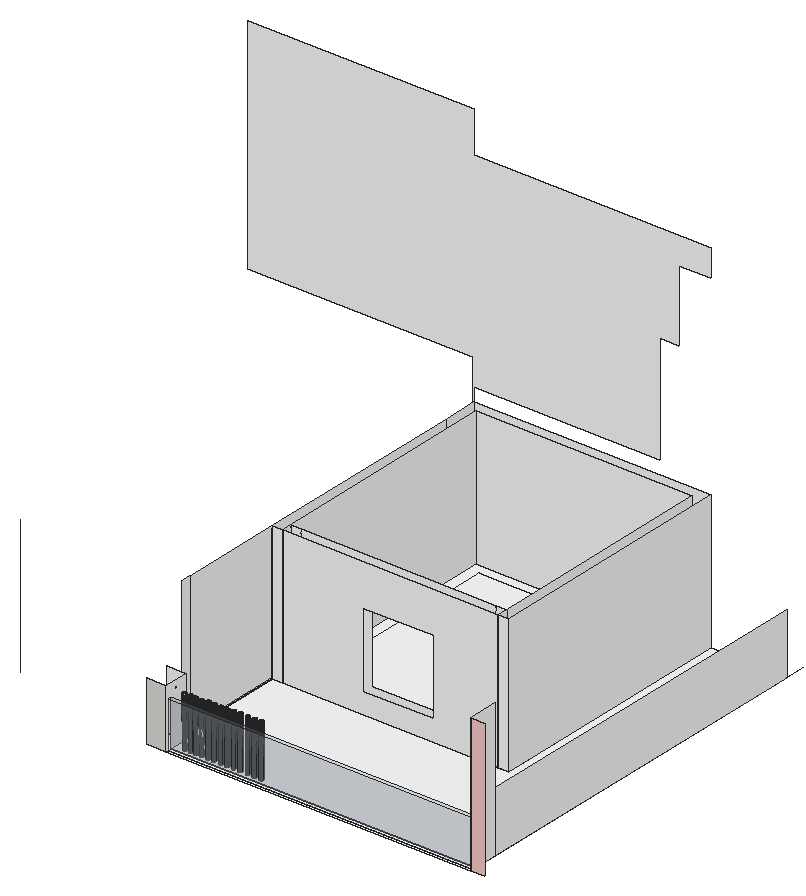
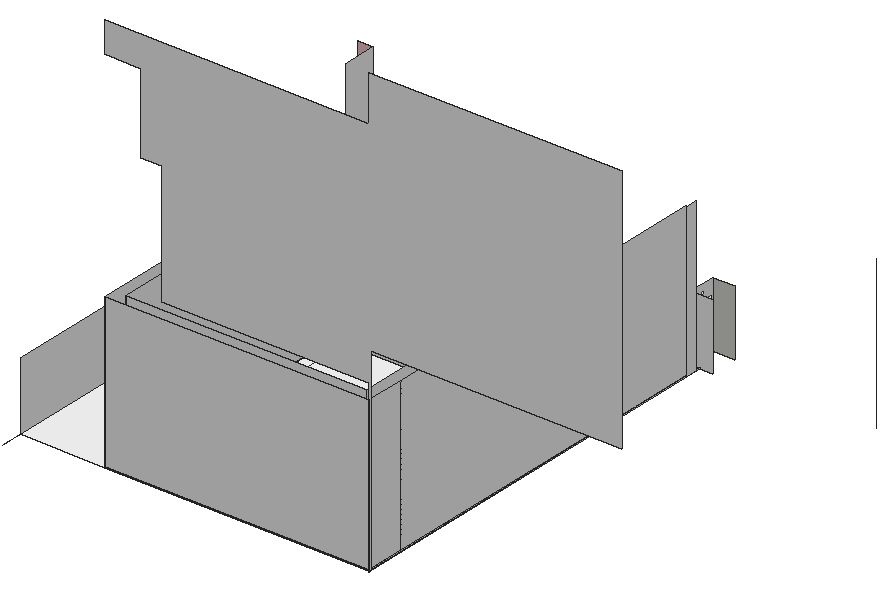
# SketchUp Ruby script. Lengths in inches.
U = 1.inch
M = Sketchup.active_model
def pt(a) = Geom::Point3d.new(a.map { |v| v * U })
def face(e, loops, mat)
  f = e.add_face(loops[0].map { |a| pt(a) })
  loops[1..].each { |l| e.add_face(l.map { |a| pt(a) }).erase! }
  f.material = f.back_material = mat if mat
  f
end
# faces: each face lists its corners as indices into pts; further lists are holes
def faces(e, pts, list, mat = nil) = list.each { |f| face(e, (f[0].is_a?(Array) ? f : [f]).map { |l| l.map { |i| pts[i] } }, mat) }
# xy, xz, yz: faces in a plane at the given z, y or x. An outline is a flat list of corners, or four numbers for a rectangle; further outlines are holes
def ring(l) = l.size == 4 ? [[l[0], l[1]], [l[2], l[1]], [l[2], l[3]], [l[0], l[3]]] : l.each_slice(2).to_a
def flat(e, list, mat, &to3) = list.each { |f| face(e, (f[0].is_a?(Array) ? f : [f]).map { |l| ring(l).map { |u, v| to3.(u, v) } }, mat) }
def xy(e, z, list, mat = nil) = flat(e, list, mat) { |x, y| [x, y, z] }
def xz(e, y, list, mat = nil) = flat(e, list, mat) { |x, z| [x, y, z] }
def yz(e, x, list, mat = nil) = flat(e, list, mat) { |y, z| [x, y, z] }
def lines(e, pts, list) = list.each { |a, b| e.add_line(pt(pts[a]), pt(pts[b])) }
# prism: a flat outline (further loops are holes) pulled along v
def prism(e, loops, v, mat = nil)
  f = face(e, loops, mat); d = Geom::Vector3d.new(v.map { |x| x * U })
  f.pushpull(f.normal.samedirection?(d) ? d.length : -d.length)
end
def box(e, o, s, mat = nil) = prism(e, [[o, [o[0] + s[0], o[1], o[2]], [o[0] + s[0], o[1] + s[1], o[2]], [o[0], o[1] + s[1], o[2]]]], [0, 0, s[2]], mat)
def at(x, y, z, deg = 0) = Geom::Transformation.translation(pt([x, y, z])) * Geom::Transformation.rotation(ORIGIN, Z_AXIS, deg.degrees)
def axes(o, x, y, z) = Geom::Transformation.new([*x, 0, *y, 0, *z, 0, *pt(o).to_a, 1])
def part(name) = M.definitions.add(name)
# library, detail: a bought-in or finely detailed component or shape, given as its bounding box
def library(name, o, s) = part(name).tap { |d| box(d.entities, o, s) }
def detail(e, o, s) = box(e.add_group.entities, o, s)
def put(e, d, t, mat = nil) = e.add_instance(d, t).tap { |i| i.material = mat if mat }
def group(e, t, mat = nil) = e.add_group.tap { |g| g.transformation = t; g.material = mat if mat }.entities
root = M.entities
M.materials.add("A01_Blush_Petal").color = [255, 204, 204]
M.materials.add("Glass_Basic_01").color = [161, 173, 186]
M.materials["Glass_Basic_01"].alpha = 0.25
M.materials.add("M00_Soft_Cloud").color = [255, 255, 255]
xy(root,264,[[205.78,136.44,472.6,138.3],[[205.78,141.64,472.6,141.64,472.6,482.39,405.98,482.39,405.98,261.09,199,261.09,199,157.97,205.78,157.97],[280.99,145.24,280.58,145.29,280.19,145.45,279.86,145.7,279.6,146.03,279.45,146.42,279.39,146.83,279.45,147.25,279.6,147.63,279.86,147.96,280.19,148.22,280.58,148.38,280.99,148.43,281.4,148.38,281.79,148.22,282.12,147.96,282.37,147.63,282.53,147.25,282.59,146.83,282.53,146.42,282.37,146.03,282.12,145.7,281.79,145.45,281.4,145.29],[256.81,145.24,256.39,145.29,256.01,145.45,255.68,145.7,255.42,146.03,255.26,146.42,255.21,146.83,255.26,147.25,255.42,147.63,255.68,147.96,256.01,148.22,256.39,148.38,256.81,148.43,257.22,148.38,257.61,148.22,257.9375,147.96,258.19,147.63,258.35,147.25,258.41,146.83,258.35,146.42,258.19,146.03,257.9375,145.7,257.61,145.45,257.22,145.29],[251.01,145.24,250.59,145.29,250.21,145.45,249.875,145.7,249.62,146.03,249.46,146.42,249.41,146.83,249.46,147.25,249.62,147.63,249.875,147.96,250.21,148.22,250.59,148.38,251.01,148.43,251.42,148.38,251.8,148.22,252.14,147.96,252.39,147.63,252.55,147.25,252.6,146.83,252.55,146.42,252.39,146.03,252.14,145.7,251.8,145.45,251.42,145.29],[245.47,145.24,245.06,145.29,244.67,145.45,244.34,145.7,244.09,146.03,243.93,146.42,243.87,146.83,243.93,147.25,244.09,147.63,244.34,147.96,244.67,148.22,245.06,148.38,245.47,148.43,245.88,148.38,246.27,148.22,246.6,147.96,246.85,147.63,247.01,147.25,247.07,146.83,247.01,146.42,246.85,146.03,246.6,145.7,246.27,145.45,245.88,145.29],[239.53,145.24,239.12,145.29,238.73,145.45,238.4,145.7,238.15,146.03,237.99,146.42,237.9375,146.83,237.99,147.25,238.15,147.63,238.4,147.96,238.73,148.22,239.12,148.38,239.53,148.43,239.95,148.38,240.33,148.22,240.66,147.96,240.92,147.63,241.08,147.25,241.13,146.83,241.08,146.42,240.92,146.03,240.66,145.7,240.33,145.45,239.95,145.29],[268.95,145.24,268.54,145.29,268.15,145.45,267.82,145.7,267.57,146.03,267.41,146.42,267.35,146.83,267.41,147.25,267.57,147.63,267.82,147.96,268.15,148.22,268.54,148.38,268.95,148.43,269.36,148.38,269.75,148.22,270.08,147.96,270.33,147.63,270.49,147.25,270.55,146.83,270.49,146.42,270.33,146.03,270.08,145.7,269.75,145.45,269.36,145.29],[262.56,145.24,262.15,145.29,261.77,145.45,261.43,145.7,261.18,146.03,261.02,146.42,260.97,146.83,261.02,147.25,261.18,147.63,261.43,147.96,261.77,148.22,262.15,148.38,262.56,148.43,262.98,148.38,263.36,148.22,263.69,147.96,263.95,147.63,264.11,147.25,264.16,146.83,264.11,146.42,263.95,146.03,263.69,145.7,263.36,145.45,262.98,145.29],[229.02,145.24,228.61,145.29,228.22,145.45,227.89,145.7,227.64,146.03,227.48,146.42,227.42,146.83,227.48,147.25,227.64,147.63,227.89,147.96,228.22,148.22,228.61,148.38,229.02,148.43,229.43,148.38,229.82,148.22,230.15,147.96,230.4,147.63,230.5625,147.25,230.62,146.83,230.5625,146.42,230.4,146.03,230.15,145.7,229.82,145.45,229.43,145.29],[223.96,145.24,223.54,145.29,223.16,145.45,222.83,145.7,222.57,146.03,222.41,146.42,222.36,146.83,222.41,147.25,222.57,147.63,222.83,147.96,223.16,148.22,223.54,148.38,223.96,148.43,224.37,148.38,224.76,148.22,225.09,147.96,225.34,147.63,225.5,147.25,225.56,146.83,225.5,146.42,225.34,146.03,225.09,145.7,224.76,145.45,224.37,145.29],[274.92,145.24,274.5,145.29,274.12,145.45,273.79,145.7,273.53,146.03,273.375,146.42,273.32,146.83,273.375,147.25,273.53,147.63,273.79,147.96,274.12,148.22,274.5,148.38,274.92,148.43,275.33,148.38,275.72,148.22,276.05,147.96,276.3,147.63,276.46,147.25,276.52,146.83,276.46,146.42,276.3,146.03,276.05,145.7,275.72,145.45,275.33,145.29],[234.29,145.24,233.875,145.29,233.49,145.45,233.16,145.7,232.9,146.03,232.74,146.42,232.6875,146.83,232.74,147.25,232.9,147.63,233.16,147.96,233.49,148.22,233.875,148.38,234.29,148.43,234.7,148.38,235.09,148.22,235.42,147.96,235.67,147.63,235.83,147.25,235.89,146.83,235.83,146.42,235.67,146.03,235.42,145.7,235.09,145.45,234.7,145.29],[219.09,145.24,218.68,145.29,218.29,145.45,217.96,145.7,217.71,146.03,217.55,146.42,217.5,146.83,217.55,147.25,217.71,147.63,217.96,147.96,218.29,148.22,218.68,148.38,219.09,148.43,219.51,148.38,219.89,148.22,220.22,147.96,220.48,147.63,220.64,147.25,220.69,146.83,220.64,146.42,220.48,146.03,220.22,145.7,219.89,145.45,219.51,145.29],[214.11,145.24,213.7,145.29,213.3125,145.45,212.98,145.7,212.73,146.03,212.57,146.42,212.51,146.83,212.57,147.25,212.73,147.63,212.98,147.96,213.3125,148.22,213.7,148.38,214.11,148.43,214.52,148.38,214.91,148.22,215.24,147.96,215.49,147.63,215.65,147.25,215.71,146.83,215.65,146.42,215.49,146.03,215.24,145.7,214.91,145.45,214.52,145.29]],[219.09,145.24,218.68,145.29,218.29,145.45,217.96,145.7,217.71,146.03,217.55,146.42,217.5,146.83,217.55,147.25,217.71,147.63,217.96,147.96,218.29,148.22,218.68,148.38,219.09,148.43,219.51,148.38,219.89,148.22,220.22,147.96,220.48,147.63,220.64,147.25,220.69,146.83,220.64,146.42,220.48,146.03,220.22,145.7,219.89,145.45,219.51,145.29],[234.29,145.24,233.875,145.29,233.49,145.45,233.16,145.7,232.9,146.03,232.74,146.42,232.6875,146.83,232.74,147.25,232.9,147.63,233.16,147.96,233.49,148.22,233.875,148.38,234.29,148.43,234.7,148.38,235.09,148.22,235.42,147.96,235.67,147.63,235.83,147.25,235.89,146.83,235.83,146.42,235.67,146.03,235.42,145.7,235.09,145.45,234.7,145.29],[245.47,145.24,245.06,145.29,244.67,145.45,244.34,145.7,244.09,146.03,243.93,146.42,243.87,146.83,243.93,147.25,244.09,147.63,244.34,147.96,244.67,148.22,245.06,148.38,245.47,148.43,245.88,148.38,246.27,148.22,246.6,147.96,246.85,147.63,247.01,147.25,247.07,146.83,247.01,146.42,246.85,146.03,246.6,145.7,246.27,145.45,245.88,145.29],
  [251.01,145.24,250.59,145.29,250.21,145.45,249.875,145.7,249.62,146.03,249.46,146.42,249.41,146.83,249.46,147.25,249.62,147.63,249.875,147.96,250.21,148.22,250.59,148.38,251.01,148.43,251.42,148.38,251.8,148.22,252.14,147.96,252.39,147.63,252.55,147.25,252.6,146.83,252.55,146.42,252.39,146.03,252.14,145.7,251.8,145.45,251.42,145.29],[199,261.09,208,261.09,208,473.39,396.98,473.39,396.98,261.09,405.98,261.09,405.98,482.39,199,482.39],[208,270.09,217,270.09,217,464.39,387.98,464.39,387.98,270.09,396.98,270.09,396.98,473.39,208,473.39],[217,270.09,387.98,464.39]],"M00_Soft_Cloud")
xy(root,264.48,[[198,162.91,199,171.91]],"M00_Soft_Cloud")
xz(root,136.44,[[189,264,205.78,315.86]])
xz(root,136.44,[[472.6,264,484.6,384]],"A01_Blush_Petal")
xz(root,138.3,[[205.78,264,472.6,304.79]],"Glass_Basic_01")
xz(root,141.64,[[205.78,264,472.6,304.79]],"Glass_Basic_01")
xz(root,157.97,[[189,263.52,189,315.86,205.78,315.86,205.78,264,199,264,199,263.52]],"M00_Soft_Cloud")
xz(root,171.91,[[198,264.48,199,384]],"M00_Soft_Cloud")
xz(root,261.09,[[199,264,208,384],[[208,264,396.98,384],[278.74,282.07,340.22,348]],[396.98,264,405.98,384]],"M00_Soft_Cloud")
xz(root,270.09,[[208,264,217,384],[[217,264,387.98,384],[278.74,282.07,340.22,348]],[387.98,264,396.98,384]],"M00_Soft_Cloud")
xz(root,473.39,[[208,264,396.98,384]],"M00_Soft_Cloud")
xz(root,482.39,[[199,264,405.98,264.48],[198,264.48,198,419.15,1,419.15,1,614.29,199,614.29,199,578.29,405.98,578.29,405.98,554.29,377.86,554.29,377.86,491.38,361.66,491.38,361.66,396,199,396,199,264.48],[199,264.48,405.98,384]],"M00_Soft_Cloud")
yz(root,198,[[162.91,264.48,171.91,384]],"M00_Soft_Cloud")
yz(root,199,[[157.97,263.52,162.91,264],[162.91,263.52,162.91,264,482.39,263.52],[482.39,263.52,162.91,264,482.39,264],[162.91,264,171.91,264.48],[171.91,264,261.09,264.48],
  [261.09,264,482.39,264.48],[171.91,264.48,261.09,384],[261.09,264.48,451.29,384],[451.29,264.48,482.39,384]],"M00_Soft_Cloud")
yz(root,205.78,[[[136.44,264,138.3,264,138.3,304.79,141.64,304.79,141.64,264,157.97,264,157.97,315.86,136.44,315.86],[147.01,308.03,146.59,308.09,146.21,308.25,145.88,308.5,145.625,308.83,145.46,309.22,145.41,309.63,145.46,310.05,145.625,310.43,145.88,310.76,146.21,311.02,146.59,311.18,147.01,311.23,147.42,311.18,147.81,311.02,148.14,310.76,148.39,310.43,148.55,310.05,148.61,309.63,148.55,309.22,148.39,308.83,148.14,308.5,147.81,308.25,147.42,308.09]]],"M00_Soft_Cloud")
yz(root,208,[[261.09,264,270.09,384],[270.09,264,473.39,384]],"M00_Soft_Cloud")
yz(root,396.98,[[261.09,264,270.09,384],[270.09,264,473.39,384]],"M00_Soft_Cloud")
yz(root,405.98,[[261.09,264,482.39,384]],"M00_Soft_Cloud")
yz(root,472.6,[[[136.44,264,136.44,384,162.91,384,162.91,264,141.64,264,141.64,304.79,138.3,304.79,138.3,264],[147.01,308.03,147.42,308.09,147.81,308.25,148.14,308.5,148.39,308.83,148.55,309.22,148.61,309.63,148.55,310.05,148.39,310.43,148.14,310.76,147.81,311.02,147.42,311.18,147.01,311.23,146.59,311.18,146.21,311.02,145.88,310.76,145.625,310.43,145.46,310.05,145.41,309.63,145.46,309.22,145.625,308.83,145.88,308.5,146.21,308.25,146.59,308.09]],[162.91,264,482.39,317.36]],"M00_Soft_Cloud")
p = [[213.7,144.08,308.79],[213.7,145.29,264],[214.11,145.24,264],[214.11,144.03,308.79],[214.52,145.29,264],[214.52,144.08,308.79],
  [223.54,144.08,308.79],[223.54,145.29,264],[223.96,145.24,264],[223.96,144.03,308.79],[224.37,145.29,264],[224.37,144.08,308.79],
  [228.61,144.08,308.79],[228.61,145.29,264],[229.02,145.24,264],[229.02,144.03,308.79],[229.43,145.29,264],[229.43,144.08,308.79],
  [213.3125,144.24,308.8],[213.3125,145.45,264],[214.91,145.45,264],[214.91,144.24,308.8],[223.16,144.24,308.8],[223.16,145.45,264],
  [224.76,145.45,264],[224.76,144.24,308.8],[228.22,144.24,308.8],[228.22,145.45,264],[229.82,145.45,264],[229.82,144.24,308.8],
  [212.98,144.49,308.8],[212.98,145.7,264],[215.24,145.7,264],[215.24,144.49,308.8],[222.83,144.49,308.8],[222.83,145.7,264],
  [225.09,145.7,264],[225.09,144.49,308.8],[227.89,144.49,308.8],[227.89,145.7,264],[230.15,145.7,264],[230.15,144.49,308.8],
  [212.73,144.83,308.8125],[212.73,146.03,264],[215.49,146.03,264],[215.49,144.83,308.8125],[222.57,144.83,308.8125],[222.57,146.03,264],
  [225.34,146.03,264],[225.34,144.83,308.8125],[227.64,144.83,308.8125],[227.64,146.03,264],[230.4,146.03,264],[230.4,144.83,308.8125],
  [212.57,145.21,308.82],[212.57,146.42,264],[215.65,146.42,264],[215.65,145.21,308.82],[222.41,145.21,308.82],[222.41,146.42,264],
  [225.5,146.42,264],[225.5,145.21,308.82],[227.48,145.21,308.82],[227.48,146.42,264],[230.5625,146.42,264],[230.5625,145.21,308.82],
  [212.51,146.83,264],[212.57,147.25,264.01],[212.73,147.63,264.02],[212.98,147.96,264.03],[213.3125,148.22,264.04],[213.7,148.375,264.04],
  [214.11,148.43,264.04],[214.52,148.375,264.04],[214.91,148.22,264.04],[215.24,147.96,264.03],[215.49,147.63,264.02],[215.65,147.25,264.01],
  [215.71,146.83,264],[215.65,146.42,263.99],[215.49,146.04,263.98],[215.24,145.7,263.97],[214.91,145.45,263.96],[214.52,145.29,263.96],
  [214.11,145.24,263.96],[213.7,145.29,263.96],[213.3125,145.45,263.96],[212.98,145.7,263.97],[212.73,146.04,263.98],[212.57,146.42,263.99],
  [212.51,145.625,308.83],[215.71,145.625,308.83],[218.68,145.29,264],[219.09,145.24,264],[219.09,145.24,308.51],[218.68,145.29,308.51],
  [219.51,145.29,264],[219.51,145.29,308.51],[222.57,146.04,263.98],[222.41,146.42,263.99],[222.36,146.83,264],[222.41,147.25,264.01],
  [222.57,147.63,264.02],[222.83,147.96,264.03],[223.16,148.22,264.04],[223.54,148.375,264.04],[223.96,148.43,264.04],[224.37,148.375,264.04],
  [224.76,148.22,264.04],[225.09,147.96,264.03],[225.34,147.63,264.02],[225.5,147.25,264.01],[225.56,146.83,264],[225.5,146.42,263.99],
  [225.34,146.04,263.98],[225.09,145.7,263.97],[224.76,145.45,263.96],[224.37,145.29,263.96],[223.96,145.24,263.96],[223.54,145.29,263.96],
  [223.16,145.45,263.96],[222.83,145.7,263.97],[222.36,145.625,308.83],[225.56,145.625,308.83],[230.4,147.63,264.02],[230.5625,147.25,264.01],
  [230.62,146.83,264],[230.5625,146.42,263.99],[230.4,146.04,263.98],[230.15,145.7,263.97],[229.82,145.45,263.96],[229.43,145.29,263.96],
  [229.02,145.24,263.96],[228.61,145.29,263.96],[228.22,145.45,263.96],[227.89,145.7,263.97],[227.64,146.04,263.98],[227.48,146.42,263.99],
  [227.42,146.83,264],[227.48,147.25,264.01],[227.64,147.63,264.02],[227.89,147.96,264.03],[228.22,148.22,264.04],[228.61,148.375,264.04],
  [229.02,148.43,264.04],[229.43,148.375,264.04],[229.82,148.22,264.04],[230.15,147.96,264.03],[227.42,145.625,308.83],[230.62,145.625,308.83],
  [233.875,145.29,264],[234.29,145.24,264],[234.29,145.24,308.83],[233.875,145.29,308.83],[234.7,145.29,264],[234.7,145.29,308.83],
  [239.12,145.29,264],[239.53,145.24,264],[239.53,145.24,308.6875],[239.12,145.29,308.6875],[239.95,145.29,264],[239.95,145.29,308.6875],
  [245.06,145.29,264],[245.47,145.24,264],[245.47,145.24,308.83],[245.06,145.29,308.83],[245.88,145.29,264],[245.88,145.29,308.83],
  [250.59,145.29,264],[251.01,145.24,264],[251.01,145.24,308.55],[250.59,145.29,308.55],[251.42,145.29,264],[251.42,145.29,308.55],
  [256.39,145.29,264],[256.81,145.24,264],[256.81,145.24,309.52],[256.39,145.29,309.52],[257.22,145.29,264],[257.22,145.29,309.52],
  [262.15,145.29,264],[262.56,145.24,264],[262.56,145.24,309.59],[262.15,145.29,309.59],[262.98,145.29,264],[262.98,145.29,309.59],
  [268.54,145.29,264],[268.95,145.24,264],[268.95,145.24,309.52],[268.54,145.29,309.52],[269.36,145.29,264],[269.36,145.29,309.52],
  [274.5,145.29,264],[274.92,145.24,264],[274.92,145.24,309.4375],[274.5,145.29,309.4375],[275.33,145.29,264],[275.33,145.29,309.4375],
  [280.58,145.29,264],[280.99,145.24,264],[280.99,145.24,309.83],[280.58,145.29,309.83],[281.4,145.29,264],[281.4,145.29,309.83],
  [218.29,145.45,264],[218.29,145.45,308.51],[219.89,145.45,264],[219.89,145.45,308.51],[233.49,145.45,264],[233.49,145.45,308.83],
  [235.09,145.45,264],[235.09,145.45,308.83],[238.73,145.45,264],[238.73,145.45,308.6875],[240.33,145.45,264],[240.33,145.45,308.6875],
  [244.67,145.45,264],[244.67,145.45,308.83],[246.27,145.45,264],[246.27,145.45,308.83],[250.21,145.45,264],[250.21,145.45,308.55],
  [251.8,145.45,264],[251.8,145.45,308.55],[256.01,145.45,264],[256.01,145.45,309.52],[257.61,145.45,264],[257.61,145.45,309.52],
  [261.77,145.45,264],[261.77,145.45,309.59],[263.36,145.45,264],[263.36,145.45,309.59],[268.15,145.45,264],[268.15,145.45,309.52],
  [269.75,145.45,264],[269.75,145.45,309.52],[274.12,145.45,264],[274.12,145.45,309.4375],[275.72,145.45,264],[275.72,145.45,309.4375],
  [280.19,145.45,264],[280.19,145.45,309.83],[281.79,145.45,264],[281.79,145.45,309.83],[217.96,145.7,264],[217.96,145.7,308.51],
  [220.22,145.7,264],[220.22,145.7,308.51],[233.16,145.7,264],[233.26,145.625,308.83],[233.16,145.7,308.83],[235.42,145.7,264],
  [235.42,145.7,308.83],[235.3125,145.625,308.83],[238.4,145.7,264],[238.4,145.7,308.6875],[240.66,145.7,264],[240.66,145.7,308.6875],
  [244.34,145.7,264],[244.44,145.625,308.83],[244.34,145.7,308.83],[246.6,145.7,264],[246.6,145.7,308.83],[246.5,145.625,308.83],
  [249.875,145.7,264],[249.875,145.7,308.55],[252.14,145.7,264],[252.14,145.7,308.55],[255.68,145.7,264],[255.68,145.7,309.52],
  [257.9375,145.7,264],[257.9375,145.7,309.52],[261.43,145.7,264],[261.43,145.7,309.59],[263.69,145.7,264],[263.69,145.7,309.59],
  [267.82,145.7,264],[267.82,145.7,309.52],[270.08,145.7,264],[270.08,145.7,309.52],[273.79,145.7,264],[273.79,145.7,309.4375],
  [276.05,145.7,264],[276.05,145.7,309.4375],[279.86,145.7,264],[279.86,145.7,309.83],[282.12,145.7,264],[282.12,145.7,309.83],
  [212.57,146.04,308.84],[215.65,146.04,308.84],[222.41,146.04,308.84],[225.5,146.04,308.84],[227.48,146.04,308.84],[230.5625,146.04,308.84],
  [217.71,146.03,264],[217.71,146.03,308.51],[220.48,146.03,264],[220.48,146.03,308.51],[232.9,146.03,264],[232.9,146.03,308.83],
  [235.67,146.03,264],[235.67,146.03,308.83],[238.15,146.03,264],[238.15,146.03,308.6875],[240.92,146.03,264],[240.92,146.03,308.6875],
  [244.09,146.03,264],[244.09,146.03,308.83],[246.85,146.03,264],[246.85,146.03,308.83],[249.62,146.03,264],[249.62,146.03,308.55],
  [252.39,146.03,264],[252.39,146.03,308.55],[255.42,146.03,264],[255.42,146.03,309.52],[258.19,146.03,264],[258.19,146.03,309.52],
  [261.18,146.03,264],[261.18,146.03,309.59],[263.95,146.03,264],[263.95,146.03,309.59],[267.57,146.03,264],[267.57,146.03,309.52],
  [270.33,146.03,264],[270.33,146.03,309.52],[273.53,146.03,264],[273.53,146.03,309.4375],[276.3,146.03,264],[276.3,146.03,309.4375],
  [279.6,146.03,264],[279.6,146.03,309.83],[282.37,146.03,264],[282.37,146.03,309.83],[212.73,146.42,308.85],[215.49,146.42,308.85],
  [217.55,146.42,264],[217.55,146.42,308.51],[220.64,146.42,264],[220.64,146.42,308.51],[222.57,146.42,308.85],[225.34,146.42,308.85],
  [227.64,146.42,308.85],[230.4,146.42,308.85],[232.74,146.42,264],[232.74,146.42,308.83],[235.83,146.42,264],[235.83,146.42,308.83],
  [237.99,146.42,264],[237.99,146.42,308.6875],[241.08,146.42,264],[241.08,146.42,308.6875],[243.93,146.42,264],[243.93,146.42,308.83],
  [247.01,146.42,264],[247.01,146.42,308.83],[249.46,146.42,264],[249.46,146.42,308.55],[252.55,146.42,264],[252.55,146.42,308.55],
  [255.26,146.42,264],[255.26,146.42,309.52],[258.35,146.42,264],[258.35,146.42,309.52],[261.02,146.42,264],[261.02,146.42,309.59],
  [264.11,146.42,264],[264.11,146.42,309.59],[267.41,146.42,264],[267.41,146.42,309.52],[270.49,146.42,264],[270.49,146.42,309.52],
  [273.375,146.42,264],[273.375,146.42,309.4375],[276.46,146.42,264],[276.46,146.42,309.4375],[279.45,146.42,264],[279.45,146.42,309.83],
  [282.53,146.42,264],[282.53,146.42,309.83],[212.98,146.75,308.86],[215.24,146.75,308.86],[217.5,146.83,264],[217.5,146.83,308.51],
  [220.69,146.83,264],[220.69,146.83,308.51],[222.83,146.75,308.86],[225.09,146.75,308.86],[227.89,146.75,308.86],[230.15,146.75,308.86],
  [232.6875,146.83,264],[232.6875,146.83,308.83],[235.89,146.83,264],[235.89,146.83,308.83],[237.9375,146.83,264],[237.9375,146.83,308.6875],
  [241.13,146.83,264],[241.13,146.83,308.6875],[243.87,146.83,264],[243.87,146.83,308.83],[247.07,146.83,264],[247.07,146.83,308.83],
  [249.41,146.83,264],[249.41,146.83,308.55],[252.6,146.83,264],[252.6,146.83,308.55],[255.21,146.83,264],[255.21,146.83,309.52],
  [258.41,146.83,264],[258.41,146.83,309.52],[260.97,146.83,264],[260.97,146.83,309.59],[264.16,146.83,264],[264.16,146.83,309.59],
  [267.35,146.83,264],[267.35,146.83,309.52],[270.55,146.83,264],[270.55,146.83,309.52],[273.32,146.83,264],[273.32,146.83,309.4375],
  [276.52,146.83,264],[276.52,146.83,309.4375],[279.39,146.83,264],[279.39,146.83,309.83],[282.59,146.83,264],[282.59,146.83,309.83],
  [213.3125,147.01,308.87],[214.91,147.01,308.87],[217.55,147.25,264],[217.55,147.25,308.51],[220.64,147.25,264],[220.64,147.25,308.51],
  [223.16,147.01,308.87],[224.76,147.01,308.87],[228.22,147.01,308.87],[229.82,147.01,308.87],[232.74,147.25,264],[232.74,147.25,308.83],
  [235.83,147.25,264],[235.83,147.25,308.83],[237.99,147.25,264],[237.99,147.25,308.6875],[241.08,147.25,264],[241.08,147.25,308.6875],
  [243.93,147.25,264],[243.93,147.25,308.83],[247.01,147.25,264],[247.01,147.25,308.83],[249.46,147.25,264],[249.46,147.25,308.55],
  [252.55,147.25,264],[252.55,147.25,308.55],[255.26,147.25,264],[255.26,147.25,309.52],[258.35,147.25,264],[258.35,147.25,309.52],
  [261.02,147.25,264],[261.02,147.25,309.59],[264.11,147.25,264],[264.11,147.25,309.59],[267.41,147.25,264],[267.41,147.25,309.52],
  [270.49,147.25,264],[270.49,147.25,309.52],[273.375,147.25,264],[273.375,147.25,309.4375],[276.46,147.25,264],[276.46,147.25,309.4375],
  [279.45,147.25,264],[279.45,147.25,309.83],[282.53,147.25,264],[282.53,147.25,309.83],[213.7,147.17,308.875],[214.52,147.17,308.875],
  [223.54,147.17,308.875],[224.37,147.17,308.875],[228.61,147.17,308.875],[229.43,147.17,308.875],[214.11,147.22,308.875],[217.71,147.63,264],
  [217.71,147.63,308.51],[220.48,147.63,264],[220.48,147.63,308.51],[223.96,147.22,308.875],[229.02,147.22,308.875],[232.9,147.63,264],
  [232.9,147.63,308.83],[235.67,147.63,264],[235.67,147.63,308.83],[238.15,147.63,264],[238.15,147.63,308.6875],[240.92,147.63,264],
  [240.92,147.63,308.6875],[244.09,147.63,264],[244.09,147.63,308.83],[246.85,147.63,264],[246.85,147.63,308.83],[249.62,147.63,264],
  [249.62,147.63,308.55],[252.39,147.63,264],[252.39,147.63,308.55],[255.42,147.63,264],[255.42,147.63,309.52],[258.19,147.63,264],
  [258.19,147.63,309.52],[261.18,147.63,264],[261.18,147.63,309.59],[263.95,147.63,264],[263.95,147.63,309.59],[267.57,147.63,264],
  [267.57,147.63,309.52],[270.33,147.63,264],[270.33,147.63,309.52],[273.53,147.63,264],[273.53,147.63,309.4375],[276.3,147.63,264],
  [276.3,147.63,309.4375],[279.6,147.63,264],[279.6,147.63,309.83],[282.37,147.63,264],[282.37,147.63,309.83],[217.96,147.96,264],
  [217.96,147.96,308.51],[220.22,147.96,264],[220.22,147.96,308.51],[233.16,147.96,264],[233.16,147.96,308.83],[235.42,147.96,264],
  [235.42,147.96,308.83],[238.4,147.96,264],[238.4,147.96,308.6875],[240.66,147.96,264],[240.66,147.96,308.6875],[244.34,147.96,264],
  [244.34,147.96,308.83],[246.6,147.96,264],[246.6,147.96,308.83],[249.875,147.96,264],[249.875,147.96,308.55],[252.14,147.96,264],
  [252.14,147.96,308.55],[255.68,147.96,264],[255.68,147.96,309.52],[257.9375,147.96,264],[257.9375,147.96,309.52],[261.43,147.96,264],
  [261.43,147.96,309.59],[263.69,147.96,264],[263.69,147.96,309.59],[267.82,147.96,264],[267.82,147.96,309.52],[270.08,147.96,264],
  [270.08,147.96,309.52],[273.79,147.96,264],[273.79,147.96,309.4375],[276.05,147.96,264],[276.05,147.96,309.4375],[279.86,147.96,264],
  [279.86,147.96,309.83],[282.12,147.96,264],[282.12,147.96,309.83],[218.29,148.22,264],[218.29,148.22,308.51],[219.89,148.22,264],
  [219.89,148.22,308.51],[233.49,148.22,264],[233.49,148.22,308.83],[235.09,148.22,264],[235.09,148.22,308.83],[238.73,148.22,264],
  [238.73,148.22,308.6875],[240.33,148.22,264],[240.33,148.22,308.6875],[244.67,148.22,264],[244.67,148.22,308.83],[246.27,148.22,264],
  [246.27,148.22,308.83],[250.21,148.22,264],[250.21,148.22,308.55],[251.8,148.22,264],[251.8,148.22,308.55],[256.01,148.22,264],
  [256.01,148.22,309.52],[257.61,148.22,264],[257.61,148.22,309.52],[261.77,148.22,264],[261.77,148.22,309.59],[263.36,148.22,264],
  [263.36,148.22,309.59],[268.15,148.22,264],[268.15,148.22,309.52],[269.75,148.22,264],[269.75,148.22,309.52],[274.12,148.22,264],
  [274.12,148.22,309.4375],[275.72,148.22,264],[275.72,148.22,309.4375],[280.19,148.22,264],[280.19,148.22,309.83],[281.79,148.22,264],
  [281.79,148.22,309.83],[218.68,148.38,264],[218.68,148.38,308.51],[219.51,148.38,264],[219.51,148.38,308.51],[233.875,148.38,264],
  [233.875,148.38,308.83],[234.7,148.38,264],[234.7,148.38,308.83],[239.12,148.38,264],[239.12,148.38,308.6875],[239.95,148.38,264],
  [239.95,148.38,308.6875],[245.06,148.38,264],[245.06,148.38,308.83],[245.88,148.38,264],[245.88,148.38,308.83],[250.59,148.38,264],
  [250.59,148.38,308.55],[251.42,148.38,264],[251.42,148.38,308.55],[256.39,148.38,264],[256.39,148.38,309.52],[257.22,148.38,264],
  [257.22,148.38,309.52],[262.15,148.38,264],[262.15,148.38,309.59],[262.98,148.38,264],[262.98,148.38,309.59],[268.54,148.38,264],
  [268.54,148.38,309.52],[269.36,148.38,264],[269.36,148.38,309.52],[274.5,148.38,264],[274.5,148.38,309.4375],[275.33,148.38,264],
  [275.33,148.38,309.4375],[280.58,148.38,264],[280.58,148.38,309.83],[281.4,148.38,264],[281.4,148.38,309.83],[219.09,148.43,264],
  [219.09,148.43,308.51],[234.29,148.43,264],[233.98,148.39,308.83],[234.29,148.43,308.83],[234.6,148.39,308.83],[239.53,148.43,264],
  [239.53,148.43,308.6875],[245.47,148.43,264],[245.16,148.39,308.83],[245.47,148.43,308.83],[245.78,148.39,308.83],[251.01,148.43,264],
  [251.01,148.43,308.55],[256.81,148.43,264],[256.81,148.43,309.52],[262.56,148.43,264],[262.56,148.43,309.59],[268.95,148.43,264],
  [268.95,148.43,309.52],[274.92,148.43,264],[274.92,148.43,309.4375],[280.99,148.43,264],[280.99,148.43,309.83],[472.6,482.39,264],
  [472.6,500.47,264],[214.11,146.83,264],[214.11,145.625,308.83],[219.09,146.83,264],[219.09,146.83,307.77],[223.96,146.83,264],
  [223.96,145.625,308.83],[234.29,146.83,264],[234.29,146.83,307.26],[239.53,146.83,264],[239.53,146.83,307.26],[245.47,146.83,264],
  [245.47,146.83,307.77],[251.01,146.83,264],[251.01,146.83,307.26],[256.81,146.83,264],[256.81,146.83,307.77],[280.99,146.83,264],
  [280.99,146.83,307.26],[274.92,146.83,264],[274.92,146.83,307.26],[268.95,146.83,264],[268.95,146.83,307.26],[262.56,146.83,264],
  [262.56,146.83,307.26],[229.02,146.83,264],[229.02,145.625,308.83],[63.09,154.91,387.8125],[63.09,154.91,267.93]]
faces(root,p,[[0,1,2,3],[3,2,4,5],[6,7,8,9],[9,8,10,11],[12,13,14,15],[15,14,16,17],[18,19,1,0],[5,4,20,21],
  [22,23,7,6],[11,10,24,25],[26,27,13,12],[17,16,28,29],[30,31,19,18],[21,20,32,33],[34,35,23,22],[25,24,36,37],
  [38,39,27,26],[29,28,40,41],[42,43,31,30],[33,32,44,45],[46,47,35,34],[37,36,48,49],[50,51,39,38],[41,40,52,53],
  [54,55,43,42],[45,44,56,57],[58,59,47,46],[49,48,60,61],[62,63,51,50],[53,52,64,65],[66,67,68,69,70,71,72,73,74,75,76,77,78,79,80,81,82,83,84,85,86,87,88,89],[90,66,55,54],
  [84,2,1,85],[83,4,2,84],[57,56,78,91],[92,93,94,95],[93,96,97,94],[98,99,100,101,102,103,104,105,106,107,108,109,110,111,112,113,114,115,116,117,118,119,120,121],[122,100,59,58],[118,8,7,119],
  [117,10,8,118],[61,60,112,123],[124,125,126,127,128,129,130,131,132,133,134,135,136,137,138,139,140,141,142,143,144,145,146,147],[148,138,63,62],[132,14,13,133],[131,16,14,132],[65,64,126,149],[150,151,152,153],
  [151,154,155,152],[156,157,158,159],[157,160,161,158],[162,163,164,165],[163,166,167,164],[168,169,170,171],[169,172,173,170],[174,175,176,177],
  [175,178,179,176],[180,181,182,183],[181,184,185,182],[186,187,188,189],[187,190,191,188],[192,193,194,195],[193,196,197,194],[198,199,200,201],
  [199,202,203,200],[85,1,19,86],[82,20,4,83],[204,92,95,205],[96,206,207,97],[119,7,23,120],[116,24,10,117],[133,13,27,134],
  [130,28,16,131],[208,150,153,209],[154,210,211,155],[212,156,159,213],[160,214,215,161],[216,162,165,217],[166,218,219,167],[220,168,171,221],
  [172,222,223,173],[224,174,177,225],[178,226,227,179],[228,180,183,229],[184,230,231,185],[232,186,189,233],[190,234,235,191],[236,192,195,237],
  [196,238,239,197],[240,198,201,241],[202,242,243,203],[86,19,31,87],[81,32,20,82],[244,204,205,245],[206,246,247,207],[120,23,35,121],
  [115,36,24,116],[134,27,39,135],[129,40,28,130],[248,208,209,249,250],[210,251,252,253,211],[254,212,213,255],[214,256,257,215],[258,216,217,259,260],
  [218,261,262,263,219],[264,220,221,265],[222,266,267,223],[268,224,225,269],[226,270,271,227],[272,228,229,273],[230,274,275,231],[276,232,233,277],
  [234,278,279,235],[280,236,237,281],[238,282,283,239],[284,240,241,285],[242,286,287,243],[67,66,90,288],[78,77,289,91],[101,100,122,290],
  [112,111,291,123],[139,138,148,292],[126,125,293,149],[87,31,43,88],[80,44,32,81],[294,244,245,295],[246,296,297,247],[121,35,47,98],
  [114,48,36,115],[135,39,51,136],[128,52,40,129],[298,248,250,299],[251,300,301,252],[302,254,255,303],[256,304,305,257],[306,258,260,307],
  [261,308,309,262],[310,264,265,311],[266,312,313,267],[314,268,269,315],[270,316,317,271],[318,272,273,319],[274,320,321,275],[322,276,277,323],
  [278,324,325,279],[326,280,281,327],[282,328,329,283],[330,284,285,331],[286,332,333,287],[88,43,55,89],[68,67,288,334],[79,56,44,80],
  [77,76,335,289],[336,294,295,337],[296,338,339,297],[98,47,59,99],[102,101,290,340],[113,60,48,114],[111,110,341,291],[136,51,63,137],
  [140,139,292,342],[127,64,52,128],[125,124,343,293],[344,298,299,345],[300,346,347,301],[348,302,303,349],[304,350,351,305],[352,306,307,353],
  [308,354,355,309],[356,310,311,357],[312,358,359,313],[360,314,315,361],[316,362,363,317],[364,318,319,365],[320,366,367,321],[368,322,323,369],
  [324,370,371,325],[372,326,327,373],[328,374,375,329],[376,330,331,377],[332,378,379,333],[89,55,66],[69,68,334,380],[76,75,381,335],
  [79,78,56],[382,336,337,383],[338,384,385,339],[99,59,100],[103,102,340,386],[110,109,387,341],[113,112,60],[137,63,138],
  [141,140,342,388],[124,147,389,343],[127,126,64],[390,344,345,391],[346,392,393,347],[394,348,349,395],[350,396,397,351],[398,352,353,399],
  [354,400,401,355],[402,356,357,403],[358,404,405,359],[406,360,361,407],[362,408,409,363],[410,364,365,411],[366,412,413,367],[414,368,369,415],
  [370,416,417,371],[418,372,373,419],[374,420,421,375],[422,376,377,423],[378,424,425,379],[70,69,380,426],[75,74,427,381],[428,382,383,429],
  [384,430,431,385],[104,103,386,432],[109,108,433,387],[142,141,388,434],[147,146,435,389],[436,390,391,437],[392,438,439,393],[440,394,395,441],
  [396,442,443,397],[444,398,399,445],[400,446,447,401],[448,402,403,449],[404,450,451,405],[452,406,407,453],[408,454,455,409],[456,410,411,457],
  [412,458,459,413],[460,414,415,461],[416,462,463,417],[464,418,419,465],[420,466,467,421],[468,422,423,469],[424,470,471,425],[71,70,426,472],
  [74,73,473,427],[105,104,432,474],[108,107,475,433],[143,142,434,476],[146,145,477,435],[72,71,472,478],[73,72,478,473],[479,428,429,480],
  [430,481,482,431],[106,105,474,483],[107,106,483,475],[144,143,476,484],[145,144,484,477],[485,436,437,486],[438,487,488,439],[489,440,441,490],
  [442,491,492,443],[493,444,445,494],[446,495,496,447],[497,448,449,498],[450,499,500,451],[501,452,453,502],[454,503,504,455],[505,456,457,506],
  [458,507,508,459],[509,460,461,510],[462,511,512,463],[513,464,465,514],[466,515,516,467],[517,468,469,518],[470,519,520,471],[521,479,480,522],
  [481,523,524,482],[525,485,486,526],[487,527,528,488],[529,489,490,530],[491,531,532,492],[533,493,494,534],[495,535,536,496],[537,497,498,538],
  [499,539,540,500],[541,501,502,542],[503,543,544,504],[545,505,506,546],[507,547,548,508],[549,509,510,550],[511,551,552,512],[553,513,514,554],
  [515,555,556,516],[557,517,518,558],[519,559,560,520],[561,521,522,562],[523,563,564,524],[565,525,526,566],[527,567,568,528],[569,529,530,570],
  [531,571,572,532],[573,533,534,574],[535,575,576,536],[577,537,538,578],[539,579,580,540],[581,541,542,582],[543,583,584,544],[585,545,546,586],
  [547,587,588,548],[589,549,550,590],[551,591,592,552],[593,553,554,594],[555,595,596,556],[597,557,558,598],[559,599,600,560],[601,561,562,602],
  [563,603,604,564],[605,565,566,606],[567,607,608,568],[609,569,570,610],[571,611,612,572],[613,573,574,614],[575,615,616,576],[617,577,578,618],
  [579,619,620,580],[621,581,582,622],[583,623,624,584],[625,585,586,626],[587,627,628,588],[629,589,590,630],[591,631,632,592],[633,593,594,634],
  [595,635,636,596],[637,597,598,638],[599,639,640,600],[641,601,602,642],[603,641,642,604],[643,605,606,644,645],[607,643,645,646,608],[647,609,610,648],
  [611,647,648,612],[649,613,614,650,651],[615,649,651,652,616],[653,617,618,654],[619,653,654,620],[655,621,622,656],[623,655,656,624],[657,625,626,658],
  [627,657,658,628],[659,629,630,660],[631,659,660,632],[661,633,634,662],[635,661,662,636],[663,637,638,664],[639,663,664,640]],"M00_Soft_Cloud")
lines(root,p,[[665,666],[667,668],[669,670],[671,672],[673,674],[675,676],[677,678],[679,680],[681,682],[683,684],[685,686],[687,688],
  [689,690],[691,692],[693,694]])
